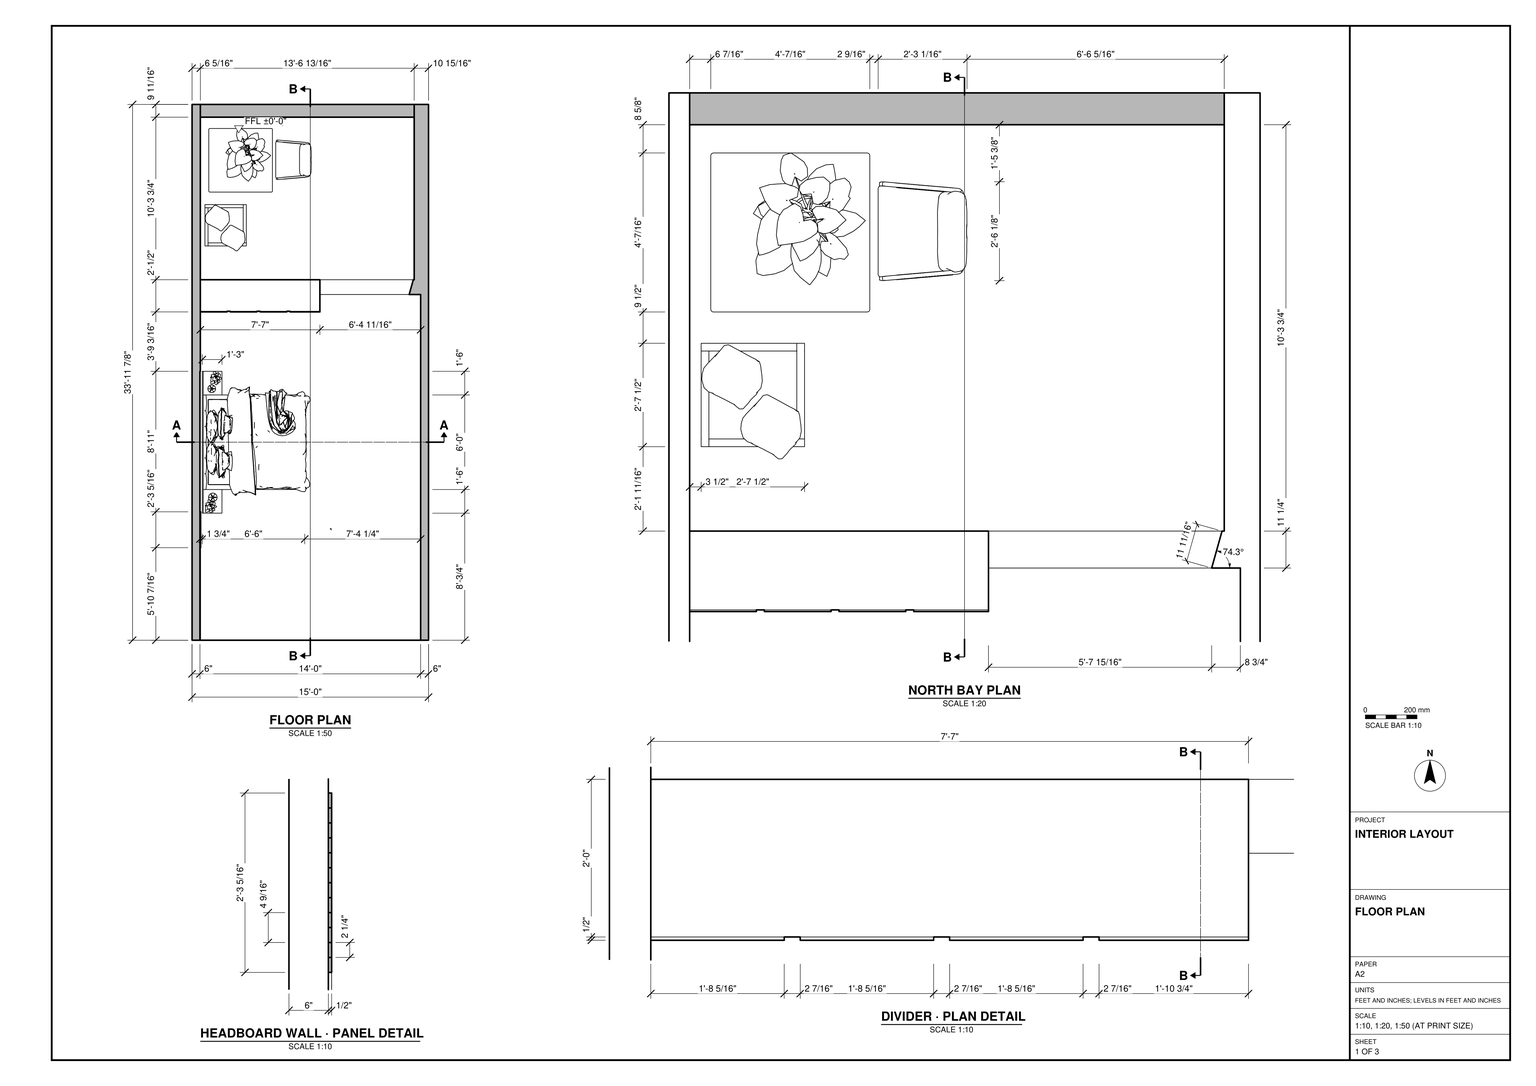
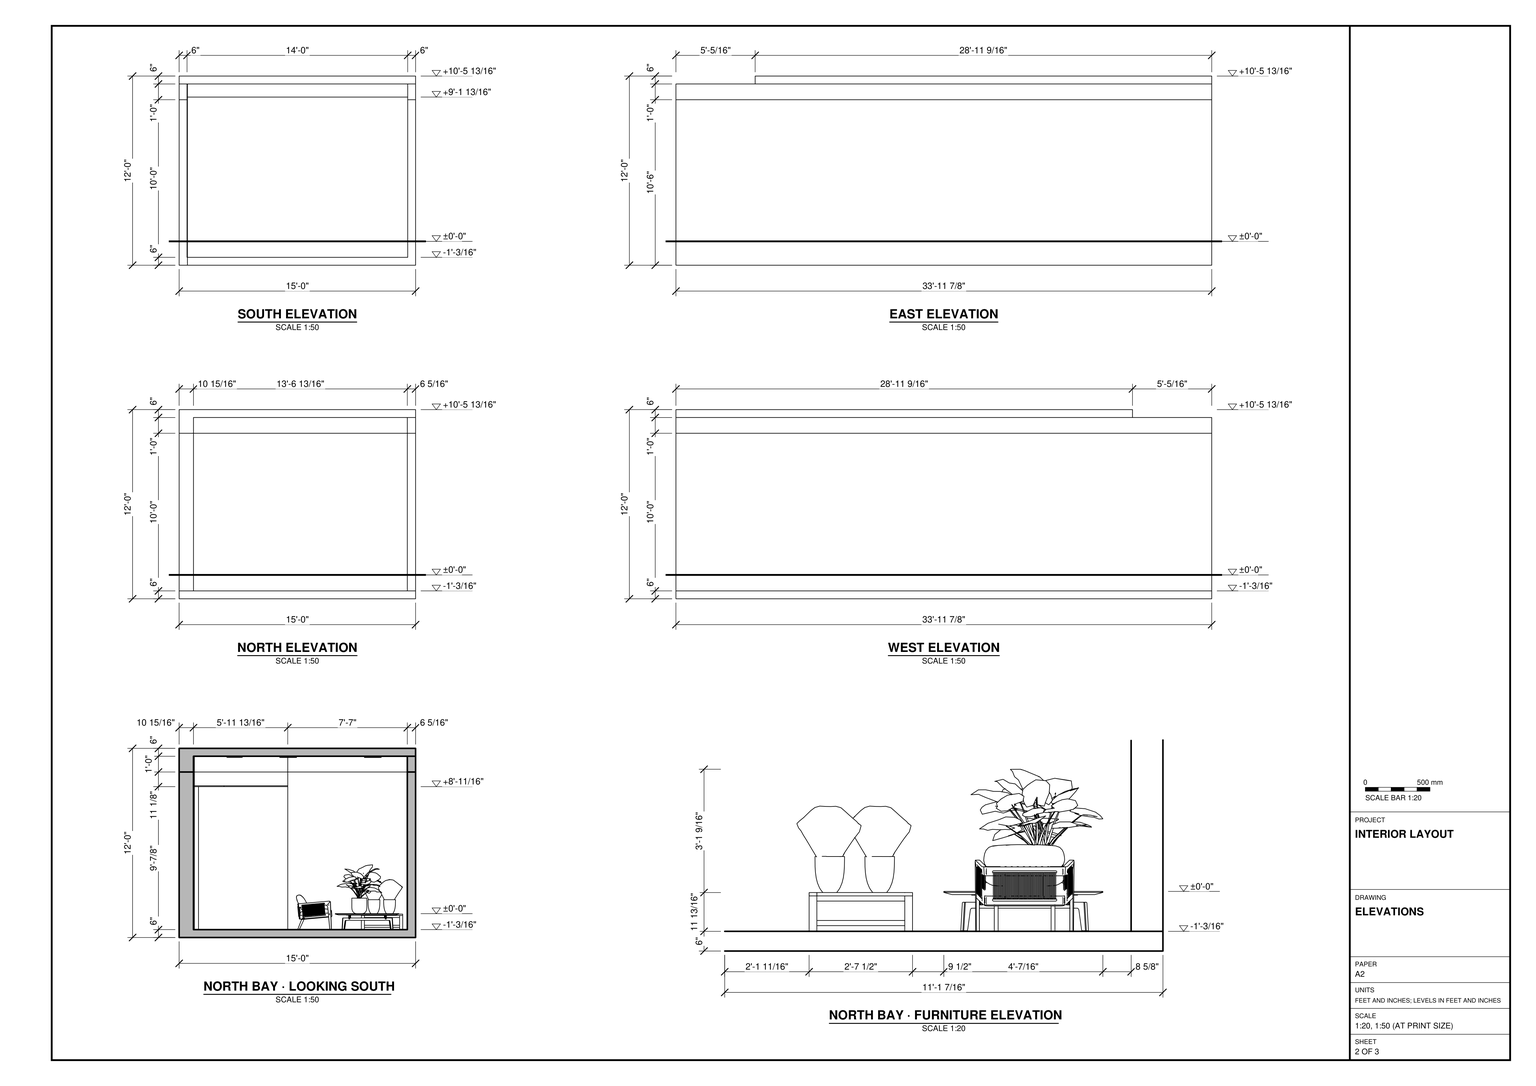
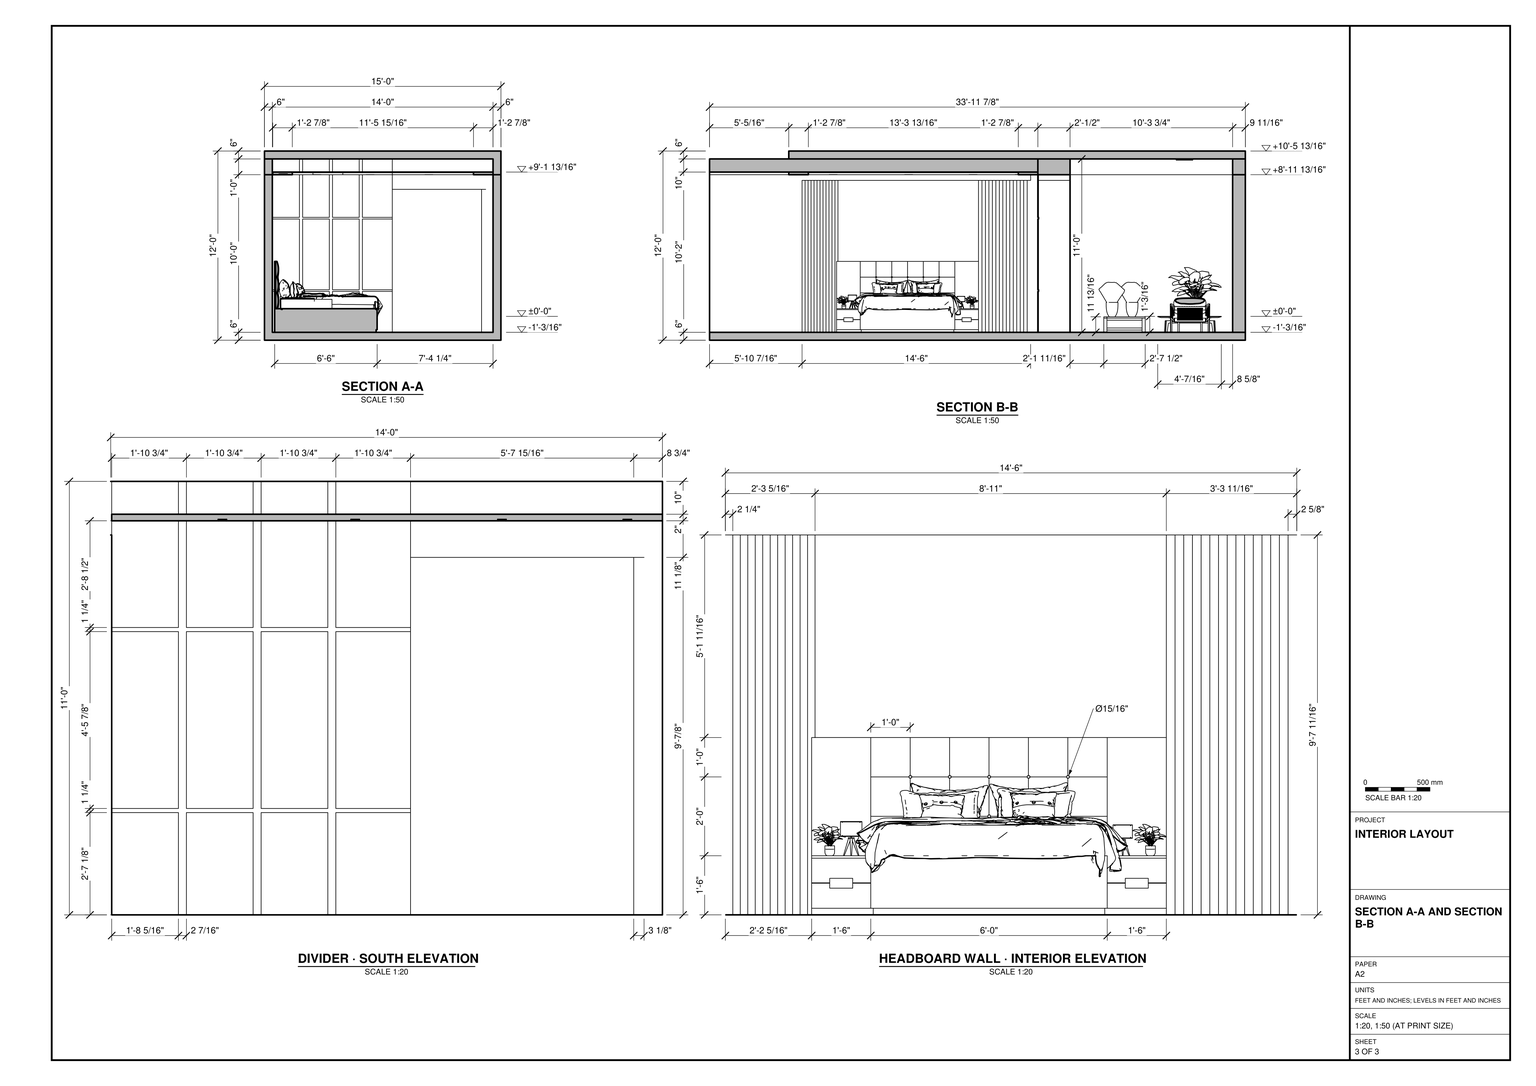
Build the furnished interior in SketchUp from task_files/diagram_01.pdf. Work in feet and inches. Set the single finished-floor datum to ±0'-0". The shell is 15'-0" wide, 33'-11 7/8" long and 12'-0" high overall. Use the floor plan for the wall footprints and thicknesses, including the angled return at the east side of the north bay. Follow the sections and exterior elevations for the floor slab, overhead slab and stepped upper profile.

Set the bed with its head against the west wall and its foot facing the clear aisle to the east. Model the bed base, mattress and paired bedside units. Use the headboard elevation to lay out the central rectangular panels and the tall, closely spaced vertical strips on either side. Between the bed and the north bay, build the divider with its panel grid facing the bed. Follow the divider plan detail for its depth and keep the passage open at its east end.

In the north bay, place the larger square low table near the northwest corner, the lounge chair to its east and the smaller square table to its south. Decor and loose items, including plants, lamps and cushions, may be any suitable library components. Keep shell elements and individual furniture and joinery pieces in separate groups or components, and use components for repeated parts. Save one SketchUp model as output_files/bedroom_with_a_panelled_divider_and_north_sitting_bay.skp.

# SketchUp Ruby script. Lengths in inches.
U = 1.inch
M = Sketchup.active_model
def pt(a) = Geom::Point3d.new(a.map { |v| v * U })
def face(e, loops, mat)
  f = e.add_face(loops[0].map { |a| pt(a) })
  loops[1..].each { |l| e.add_face(l.map { |a| pt(a) }).erase! }
  f.material = f.back_material = mat if mat
  f
end
# faces: each face lists its corners as indices into pts; further lists are holes
def faces(e, pts, list, mat = nil) = list.each { |f| face(e, (f[0].is_a?(Array) ? f : [f]).map { |l| l.map { |i| pts[i] } }, mat) }
# xy, xz, yz: faces in a plane at the given z, y or x. An outline is a flat list of corners, or four numbers for a rectangle; further outlines are holes
def ring(l) = l.size == 4 ? [[l[0], l[1]], [l[2], l[1]], [l[2], l[3]], [l[0], l[3]]] : l.each_slice(2).to_a
def flat(e, list, mat, &to3) = list.each { |f| face(e, (f[0].is_a?(Array) ? f : [f]).map { |l| ring(l).map { |u, v| to3.(u, v) } }, mat) }
def xy(e, z, list, mat = nil) = flat(e, list, mat) { |x, y| [x, y, z] }
def xz(e, y, list, mat = nil) = flat(e, list, mat) { |x, z| [x, y, z] }
def yz(e, x, list, mat = nil) = flat(e, list, mat) { |y, z| [x, y, z] }
def lines(e, pts, list) = list.each { |a, b| e.add_line(pt(pts[a]), pt(pts[b])) }
# prism: a flat outline (further loops are holes) pulled along v
def prism(e, loops, v, mat = nil)
  f = face(e, loops, mat); d = Geom::Vector3d.new(v.map { |x| x * U })
  f.pushpull(f.normal.samedirection?(d) ? d.length : -d.length)
end
def box(e, o, s, mat = nil) = prism(e, [[o, [o[0] + s[0], o[1], o[2]], [o[0] + s[0], o[1] + s[1], o[2]], [o[0], o[1] + s[1], o[2]]]], [0, 0, s[2]], mat)
def at(x, y, z, deg = 0) = Geom::Transformation.translation(pt([x, y, z])) * Geom::Transformation.rotation(ORIGIN, Z_AXIS, deg.degrees)
def axes(o, x, y, z) = Geom::Transformation.new([*x, 0, *y, 0, *z, 0, *pt(o).to_a, 1])
def part(name) = M.definitions.add(name)
# library, detail: a bought-in or finely detailed component or shape, given as its bounding box
def library(name, o, s) = part(name).tap { |d| box(d.entities, o, s) }
def detail(e, o, s) = box(e.add_group.entities, o, s)
def put(e, d, t, mat = nil) = e.add_instance(d, t).tap { |i| i.material = mat if mat }
def group(e, t, mat = nil) = e.add_group.tap { |g| g.transformation = t; g.material = mat if mat }.entities
root = M.entities
M.materials.add("Emissive").color = [250, 245, 210]
M.materials.add("Generic").color = [222, 222, 222]
M.materials.add("Tiles Marble White 03 180cm").color = [26, 26, 26]
M.materials.add("[0043_SaddleBrown]").color = [139, 69, 19]
M.materials.add("[0052_FloralWhite]").color = [119, 119, 119]
M.materials.add("[0129_WhiteSmoke]").color = [244, 244, 244]
M.materials.add("[Color B08]").color = [102, 25, 0]
M.materials.add("[Color C08]").color = [102, 51, 0]
M.materials.add("[Color M00]").color = [255, 255, 255]
M.materials.add("[Wood Veneer 01]").color = [120, 70, 37]
c1 = library("Untitled (3)",[0,0,0],[120.78,98.35,54])
c2 = library("poliform+coffee+table+TRIBECA",[0.44,0,0],[48.42,48.43,12.17])
c3 = library("RRLC03",[0,0,0],[27.06,30.13,26.4])
c4 = library("Table Coffee 97-30",[-15.75,-15.75,0],[31.5,31.5,11.8125])
c5 = library("Sansevieria 001",[-9.82,-9.99,0],[18.42,19.55,26.33])
c6 = library("Indoor Plant 001",[-24.46,-30.5625,0],[48.74,57.4,53.14])
c7 = library("Tlon Light 1350 Ceiling 152 009",[-26.57,-26.57,-3.78],[53.14,53.14,3.72])
c8 = library("Lamp Table 114-28",[-7.97,-7.97,0],[15.94,15.94,25.4375])
xy(root,-6,[[0,0,180,407.875]])
xy(root,0,[[6,0,6.5,70.4375],[6,70.4375,6.5,72.71],[6,72.71,6.5,74.99],[6,74.99,6.5,77.27],[6,77.27,6.5,79.54],
  [6,79.54,6.5,81.82],[6,81.82,6.5,84.09],[6,84.09,6.5,86.37],[6,86.37,6.5,88.65],[6,88.65,6.5,90.92],
  [6,90.92,6.5,93.2],[6,93.2,6.5,95.47],[6,95.47,6.5,97.75],[6.3,249.9375,6.3,274.4375,97.3,274.4375,97.3,249.9375,74.55,249.9375,74.55,250.4375,72.11,250.4375,72.11,249.9375,51.8,249.9375,51.8,250.4375,49.36,250.4375,49.36,249.9375,29.05,249.9375,29.05,250.4375,26.61,250.4375,26.61,249.9375],[6.3,398.1875,169.09,407.875]])
xy(root,0,[[6.5,0,6.5,97.75,6,97.75,6,204.72,6.3,204.72,6.3,249.9375,26.61,249.9375,26.61,250.4375,29.05,250.4375,29.05,249.9375,49.36,249.9375,49.36,250.4375,51.8,250.4375,51.8,249.9375,72.11,249.9375,72.11,250.4375,74.55,250.4375,74.55,249.9375,97.3,249.9375,97.3,263.1875,174,263.1875,174,0],[6.3,274.4375,169.09,398.1875]],"Tiles Marble White 03 180cm")
xy(root,0,[[97.3,263.1875,97.3,274.4375,168.41,274.4375,165.26,263.1875]],"[Wood Veneer 01]")
xy(root,31.14,[[6.3,249.9375,26.61,250.4375],[29.05,249.9375,49.36,250.4375],[51.8,249.9375,72.11,250.4375],[74.55,249.9375,97.3,250.4375]])
xy(root,32.39,[[6.3,249.9375,26.61,250.4375],[29.05,249.9375,49.36,250.4375],[51.8,249.9375,72.11,250.4375],[74.55,249.9375,97.3,250.4375]])
xy(root,86.25,[[6.3,249.9375,26.61,250.4375],[29.05,249.9375,49.36,250.4375],[51.8,249.9375,72.11,250.4375],[74.55,249.9375,97.3,250.4375]])
xy(root,87.51,[[6.3,249.9375,26.61,250.4375],[29.05,249.9375,49.36,250.4375],[51.8,249.9375,72.11,250.4375],[74.55,249.9375,97.3,250.4375]])
xy(root,108.86,[[165.26,263.1875,168.41,274.4375,168.41,263.1875]])
xy(root,108.86,[[97.3,263.1875,97.3,274.4375,168.41,274.4375,165.26,263.1875]],"[Color C08]")
xy(root,115.6875,[[6,204.72,6.3,207.37],[6,207.37,6.3,210.02],[6,210.02,6.3,212.67],[6,212.67,6.3,215.3125],[6,215.3125,6.3,217.96],
  [6,217.96,6.3,220.61],[6,220.61,6.3,223.26],[6,223.26,6.3,225.9],[6,225.9,6.3,228.55],[6,228.55,6.3,231.2],
  [6,231.2,6.3,233.85],[6,233.85,6.3,236.49],[6,236.49,6.3,239.14],[6,239.14,6.3,241.79]])
xy(root,115.6875,[[6,70.4375,6.5,72.71],[6,72.71,6.5,74.99],[6,74.99,6.5,77.27],[6,77.27,6.5,79.54],[6,79.54,6.5,81.82],
  [6,81.82,6.5,84.09],[6,84.09,6.5,86.37],[6,86.37,6.5,88.65],[6,88.65,6.5,90.92],[6,90.92,6.5,93.2],
  [6,93.2,6.5,95.47],[6,95.47,6.5,97.75]],"[0043_SaddleBrown]")
xy(root,115.6875,[[6,241.79,6.3,244.4375]],"[0129_WhiteSmoke]")
xy(root,120,[[[0,0,0,407.875,180,407.875,180,0,174,0,174,263.1875,97.3,263.1875,97.3,249.9375,74.55,249.9375,74.55,250.4375,72.11,250.4375,72.11,249.9375,51.8,249.9375,51.8,250.4375,49.36,250.4375,49.36,249.9375,29.05,249.9375,29.05,250.4375,26.61,250.4375,26.61,249.9375,6.3,249.9375,6.3,244.4375,6,244.4375,6,0],[6.3,274.4375,169.09,398.1875]]],"[Color M00]")
xy(root,122,[[6,0,174,60.3125]])
xy(root,132,[[6,0,6.3,60.3125],[6.3,0,174,60.3125],[6,60.3125,6.3,244.4375],[6.3,60.3125,6.3,249.9375,26.61,249.9375,26.61,250.4375,29.05,250.4375,29.05,249.9375,49.36,249.9375,49.36,250.4375,51.8,250.4375,51.8,249.9375,72.11,249.9375,72.11,250.4375,74.55,250.4375,74.55,249.9375,174,249.9375,174,60.3125],[97.3,249.9375,174,263.1875],
  [6.3,274.4375,169.09,398.1875]])
xy(root,132,[[0,0,6,60.3125],[174,0,180,60.3125],[0,60.3125,6,60.3125,6,244.4375,6.3,244.4375,6.3,407.875,0,407.875],[6.3,249.9375,26.61,249.9375,26.61,250.4375,29.05,250.4375,29.05,249.9375,49.36,249.9375,49.36,250.4375,51.8,250.4375,51.8,249.9375,72.11,249.9375,72.11,250.4375,74.55,250.4375,74.55,249.9375,97.3,249.9375,97.3,263.1875,169.09,263.1875,169.09,274.4375,6.3,274.4375],[6.3,398.1875,169.09,407.875]],"[Color M00]")
xy(root,138,[[0,60.3125,180,407.875]])
xz(root,0,[[0,-6,6.3,-6,6.3,0,6,0,6,120,0,120],[6.3,-6,180,-6,180,120,174,120,174,0,6.3,0],[6,0,6.3,122],[6.3,0,174,122],[6,122,6.3,132],
  [6.3,122,174,132]])
xz(root,0,[[0,120,6,132],[174,120,180,132]],"[Color M00]")
xz(root,60.3125,[[0,132,180,138]])
xz(root,70.4375,[[6,0,6.5,115.6875]],"[0043_SaddleBrown]")
xz(root,72.71,[[6,0,6.5,115.6875]])
xz(root,74.99,[[6,0,6.5,115.6875]])
xz(root,77.27,[[6,0,6.5,115.6875]])
xz(root,79.54,[[6,0,6.5,115.6875]])
xz(root,81.82,[[6,0,6.5,115.6875]])
xz(root,84.09,[[6,0,6.5,115.6875]])
xz(root,86.37,[[6,0,6.5,115.6875]])
xz(root,88.65,[[6,0,6.5,115.6875]])
xz(root,90.92,[[6,0,6.5,115.6875]])
xz(root,93.2,[[6,0,6.5,115.6875]])
xz(root,95.47,[[6,0,6.5,115.6875]])
xz(root,97.75,[[6,0,6.5,115.6875]],"[0043_SaddleBrown]")
xz(root,204.72,[[6,0,6.3,115.6875]])
xz(root,244.4375,[[6,115.6875,6.3,120]])
xz(root,244.4375,[[6,120,6.3,132]],"[Color M00]")
xz(root,249.9375,[[6.3,0,26.61,31.14],[29.05,0,49.36,31.14],[51.8,0,72.11,31.14],[74.55,0,97.3,31.14],[6.3,32.39,26.61,86.25],
  [29.05,32.39,49.36,86.25],[51.8,32.39,72.11,86.25],[74.55,32.39,97.3,86.25],[6.3,87.51,26.61,120],[29.05,87.51,49.36,120],
  [51.8,87.51,72.11,120],[74.55,87.51,97.3,120]],"Generic")
xz(root,249.9375,[[6.3,120,26.61,132],[29.05,120,49.36,132],[51.8,120,72.11,132],[74.55,120,97.3,132]],"[Color M00]")
xz(root,250.4375,[[72.11,0,74.55,31.14],[72.11,31.14,74.55,32.39],[74.55,31.14,97.3,32.39]],"[Color B08]")
xz(root,250.4375,[[[26.61,0,29.05,0,29.05,31.14,49.36,31.14,49.36,0,51.8,0,51.8,31.14,72.11,31.14,72.11,32.39,51.8,32.39,51.8,86.25,72.11,86.25,72.11,32.39,74.55,32.39,74.55,86.25,97.3,86.25,97.3,87.51,74.55,87.51,74.55,120,72.11,120,72.11,87.51,51.8,87.51,51.8,120,49.36,120,49.36,87.51,29.05,87.51,29.05,120,26.61,120,26.61,87.51,6.3,87.51,6.3,86.25,26.61,86.25,26.61,32.39,6.3,32.39,6.3,31.14,26.61,31.14],[29.05,32.39,49.36,86.25]]],"[Color C08]")
xz(root,250.4375,[[26.61,120,29.05,132],[49.36,120,51.8,132],[72.11,120,74.55,132]],"[Color M00]")
xz(root,263.1875,[[97.3,120,174,132]],"[Color M00]")
xz(root,263.1875,[[165.26,0,174,0,174,120,97.3,120,97.3,108.86,165.26,108.86]],"[Wood Veneer 01]")
xz(root,274.4375,[[6.3,0,97.3,120],[168.41,0,169.09,120],[145.86,108.86,168.41,109.51],[97.3,109.51,168.41,120]])
xz(root,274.4375,[[97.3,108.86,145.86,109.51]],"[Color C08]")
xz(root,274.4375,[[6.3,120,97.3,132],[97.3,120,168.41,132],[168.41,120,169.09,132]],"[Color M00]")
xz(root,398.1875,[[6.3,0,169.09,120],[6.3,120,169.09,132]],"[Color M00]")
xz(root,407.875,[[0,-6,180,0],[0,0,6.3,120],[6.3,0,169.09,120],[169.09,0,180,120],[169.09,120,169.09,132,0,132,0,138,180,138,180,120]])
xz(root,407.875,[[0,120,6.3,132],[6.3,120,169.09,132]],"[Color M00]")
yz(root,0,[[0,-6,407.875,0],[0,0,407.875,120],[60.3125,132,407.875,138]])
yz(root,0,[[0,120,407.875,132]],"[Color M00]")
yz(root,6,[[70.4375,0,72.71,115.6875],[72.71,0,74.99,115.6875],[74.99,0,77.27,115.6875],[77.27,0,79.54,115.6875],[79.54,0,81.82,115.6875],
  [81.82,0,84.09,115.6875],[84.09,0,86.37,115.6875],[86.37,0,88.65,115.6875],[88.65,0,90.92,115.6875],[90.92,0,93.2,115.6875],
  [93.2,0,95.47,115.6875],[95.47,0,97.75,115.6875],[97.75,0,204.72,115.6875]])
yz(root,6,[[0,0,70.4375,0,70.4375,115.6875,244.4375,115.6875,244.4375,120,0,120]],"[0052_FloralWhite]")
yz(root,6,[[0,120,244.4375,132]],"[Color M00]")
yz(root,6.3,[[249.9375,0,274.4375,0,274.4375,115.6875,249.9375,115.6875,249.9375,87.51,250.4375,87.51,250.4375,86.25,249.9375,86.25,249.9375,32.39,250.4375,32.39,250.4375,31.14,249.9375,31.14],[274.4375,0,398.1875,120],[398.1875,0,407.875,132]])
yz(root,6.3,[[204.72,0,207.37,115.6875],[207.37,0,210.02,115.6875],[210.02,0,212.67,115.6875],[212.67,0,215.3125,115.6875],[215.3125,0,217.96,115.6875],
  [217.96,0,220.61,115.6875],[220.61,0,223.26,115.6875],[223.26,0,225.9,115.6875],[225.9,0,228.55,115.6875],[228.55,0,231.2,115.6875],
  [231.2,0,233.85,115.6875],[233.85,0,236.49,115.6875],[236.49,0,239.14,115.6875],[239.14,0,241.79,115.6875]],"[0043_SaddleBrown]")
yz(root,6.3,[[241.79,0,249.9375,0,249.9375,31.14,250.4375,31.14,250.4375,32.39,249.9375,32.39,249.9375,86.25,250.4375,86.25,250.4375,87.51,249.9375,87.51,249.9375,120,244.4375,120,244.4375,115.6875,241.79,115.6875]],"[0129_WhiteSmoke]")
yz(root,6.3,[[244.4375,120,249.9375,132],[274.4375,120,398.1875,132]],"[Color M00]")
yz(root,6.5,[[70.4375,0,72.71,115.6875],[72.71,0,74.99,115.6875],[74.99,0,77.27,115.6875],[77.27,0,79.54,115.6875],[79.54,0,81.82,115.6875],
  [81.82,0,84.09,115.6875],[84.09,0,86.37,115.6875],[86.37,0,88.65,115.6875],[88.65,0,90.92,115.6875],[90.92,0,93.2,115.6875],
  [93.2,0,95.47,115.6875],[95.47,0,97.75,115.6875]],"[0043_SaddleBrown]")
yz(root,26.61,[[249.9375,0,250.4375,31.14],[249.9375,32.39,250.4375,86.25],[249.9375,87.51,250.4375,120]])
yz(root,26.61,[[249.9375,120,250.4375,132]],"[Color M00]")
yz(root,29.05,[[249.9375,0,250.4375,31.14],[249.9375,32.39,250.4375,86.25],[249.9375,87.51,250.4375,120]])
yz(root,29.05,[[249.9375,120,250.4375,132]],"[Color M00]")
yz(root,49.36,[[249.9375,0,250.4375,31.14],[249.9375,32.39,250.4375,86.25],[249.9375,87.51,250.4375,120]])
yz(root,49.36,[[249.9375,120,250.4375,132]],"[Color M00]")
yz(root,51.8,[[249.9375,0,250.4375,31.14],[249.9375,32.39,250.4375,86.25],[249.9375,87.51,250.4375,120]])
yz(root,51.8,[[249.9375,120,250.4375,132]],"[Color M00]")
yz(root,72.11,[[249.9375,0,250.4375,31.14],[249.9375,32.39,250.4375,86.25],[249.9375,87.51,250.4375,120]])
yz(root,72.11,[[249.9375,120,250.4375,132]],"[Color M00]")
yz(root,74.55,[[249.9375,0,250.4375,31.14],[249.9375,32.39,250.4375,86.25],[249.9375,87.51,250.4375,120]])
yz(root,74.55,[[249.9375,120,250.4375,132]],"[Color M00]")
yz(root,97.3,[[263.1875,108.86,274.4375,115.6875]],"[Color C08]")
yz(root,97.3,[[249.9375,120,263.1875,132]],"[Color M00]")
yz(root,97.3,[[249.9375,0,274.4375,0,274.4375,108.86,263.1875,108.86,263.1875,120,249.9375,120,249.9375,87.51,250.4375,87.51,250.4375,86.25,249.9375,86.25,249.9375,32.39,250.4375,32.39,250.4375,31.14,249.9375,31.14]],"[Wood Veneer 01]")
yz(root,169.09,[[274.4375,0,398.1875,120],[398.1875,0,407.875,132]])
yz(root,169.09,[[274.4375,120,398.1875,132]],"[Color M00]")
yz(root,174,[[0,0,263.1875,120]])
yz(root,174,[[0,120,263.1875,132]],"[Color M00]")
yz(root,180,[[0,-6,407.875,120],[60.3125,132,407.875,138]])
yz(root,180,[[0,120,407.875,132]],"[Color M00]")
p = [[165.26,263.1875,108.86],[168.41,274.4375,108.86],[168.41,274.4375,0],[165.26,263.1875,0],[51.8,250.4375,87.5],[51.8,250.4375,87.51],
  [72.11,250.4375,87.5],[72.11,250.4375,87.51]]
faces(root,p,[[0,1,2,3]],"[Color C08]")
lines(root,p,[[4,5],[6,7]])
put(root,c1,at(106.1,83.9375,0,90))
put(root,c2,at(12.3,341.16,0))
put(root,c3,at(90.75,380.82,0,180))
put(root,c4,at(25.55,315.88,0))
put(root,c5,at(19.8125,321.62,11.8125))
put(root,c5,at(31.69,306.41,11.8125))
put(root,c6,axes([42.83,370.79,12.17],[0.7,0,0],[0,0.7,0],[0,0,0.7]))
put(root,c7,axes([137.79,358.79,131.95],[0.22,0,0],[0,0.22,0],[0,0,0.22]))
put(root,c7,axes([32.58,361.53,131.96],[0.24,0,0],[0,0.24,0],[0,0,0.24]))
put(root,c7,axes([97.02,361.53,131.96],[0.24,0,0],[0,0.24,0],[0,0,0.24]))
put(root,c8,axes([15.79,108.76,18],[0.41,0,0],[0,0.41,0],[0,0,0.41]))
put(root,c8,axes([14.96,191.43,18],[0.37,0,0],[0,0.37,0],[0,0,0.37]))
put(root,c6,axes([14.35,102.22,18],[0.18,0,0],[0,0.18,0],[0,0,0.18]))
put(root,c6,axes([18.39,199.89,18],[0.18,0,0],[0,0.18,0],[0,0,0.18]))
g1 = group(root,at(6.3,60.3125,119.99))
xy(g1,0.01,[[[0,0,0,189.625,20.3125,189.625,20.3125,190.125,22.75,190.125,22.75,189.625,43.0625,189.625,43.0625,190.125,45.5,190.125,45.5,189.625,65.8125,189.625,65.8125,190.125,68.25,190.125,68.25,189.625,167.7,189.625,167.7,0],[14.89,14.89,152.81,174.73]]])
xy(g1,1.83,[[14.89,14.89,152.81,174.73]])
xy(g1,2.01,[[0,0,167.7,0,167.7,189.625,68.25,189.625,68.25,190.125,65.8125,190.125,65.8125,189.625,45.5,189.625,45.5,190.125,43.0625,190.125,43.0625,189.625,22.75,189.625,22.75,190.125,20.3125,190.125,20.3125,189.625,0,189.625]])
xz(g1,0,[[0,0.01,167.7,2.01]])
xz(g1,14.89,[[14.89,0.01,152.81,1.83]],"Emissive")
xz(g1,174.73,[[14.89,0.01,30.61,1.83],[30.61,0.01,53.36,1.83],[53.36,0.01,91,1.83],[91,0.01,152.81,1.83]],"Emissive")
xz(g1,189.625,[[0,0.01,20.3125,2.01],[22.75,0.01,43.0625,2.01],[45.5,0.01,65.8125,2.01],[68.25,0.01,91,2.01],[91,0.01,167.7,2.01]])
xz(g1,190.125,[[20.3125,0.01,22.75,2.01],[43.0625,0.01,45.5,2.01],[65.8125,0.01,68.25,2.01]])
yz(g1,0,[[0,0.01,184.125,2.01],[184.125,0.01,189.625,2.01]])
yz(g1,14.89,[[14.89,0.01,174.73,1.83]],"Emissive")
yz(g1,20.3125,[[189.625,0.01,190.125,2.01]])
yz(g1,22.75,[[189.625,0.01,190.125,2.01]])
yz(g1,43.0625,[[189.625,0.01,190.125,2.01]])
yz(g1,45.5,[[189.625,0.01,190.125,2.01]])
yz(g1,65.8125,[[189.625,0.01,190.125,2.01]])
yz(g1,68.25,[[189.625,0.01,190.125,2.01]])
yz(g1,152.81,[[14.89,0.01,174.73,1.83]],"Emissive")
yz(g1,167.7,[[0,0.01,189.625,2.01]])
put(g1,c7,axes([7.76,140.3125,0.47],[0.12,0,0],[0,0.12,0],[0,0,0.12]))
put(g1,c7,axes([7.95,91.25,0.47],[0.12,0,0],[0,0.12,0],[0,0,0.12]))
put(g1,c7,axes([7.95,33.8125,0.47],[0.12,0,0],[0,0.12,0],[0,0,0.12]))
put(g1,c7,axes([118.83,182.66,0.45],[0.12,0,0],[0,0.12,0],[0,0,0.12]))
put(g1,c7,axes([157.02,182.66,0.45],[0.12,0,0],[0,0.12,0],[0,0,0.12]))
put(g1,c7,axes([157.02,139.77,0.45],[0.12,0,0],[0,0.12,0],[0,0,0.12]))
put(g1,c7,axes([74.14,182.66,0.45],[0.12,0,0],[0,0.12,0],[0,0,0.12]))
put(g1,c7,axes([33.7,182.66,0.45],[0.12,0,0],[0,0.12,0],[0,0,0.12]))
put(g1,c7,axes([7.76,175.375,0.47],[0.12,0,0],[0,0.12,0],[0,0,0.12]))
put(g1,c7,axes([53.58,11.1,0.45],[0.12,0,0],[0,0.12,0],[0,0,0.12]))
put(g1,c7,axes([157.02,96.88,0.45],[0.12,0,0],[0,0.12,0],[0,0,0.12]))
put(g1,c7,axes([157.02,53.99,0.45],[0.12,0,0],[0,0.12,0],[0,0,0.12]))
put(g1,c7,axes([157.02,11.1,0.45],[0.12,0,0],[0,0.12,0],[0,0,0.12]))
put(g1,c7,axes([101.89,11.1,0.45],[0.12,0,0],[0,0.12,0],[0,0,0.12]))
put(g1,c7,axes([11.77,11.1,0.45],[0.12,0,0],[0,0.12,0],[0,0,0.12]))
